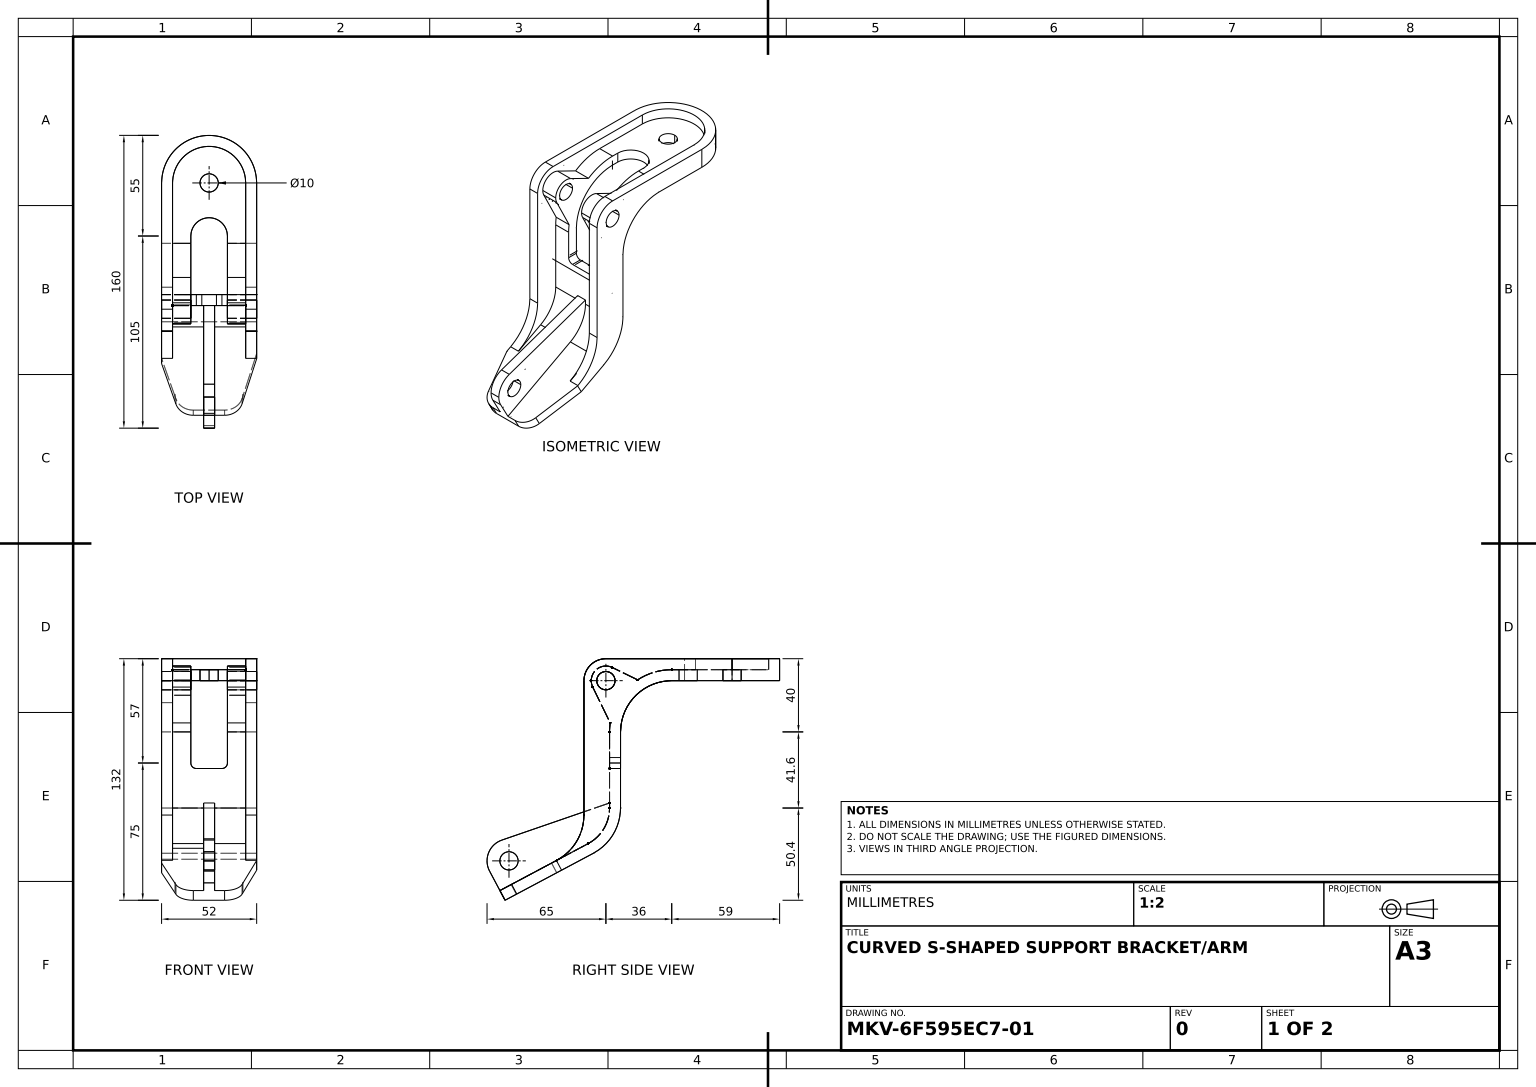
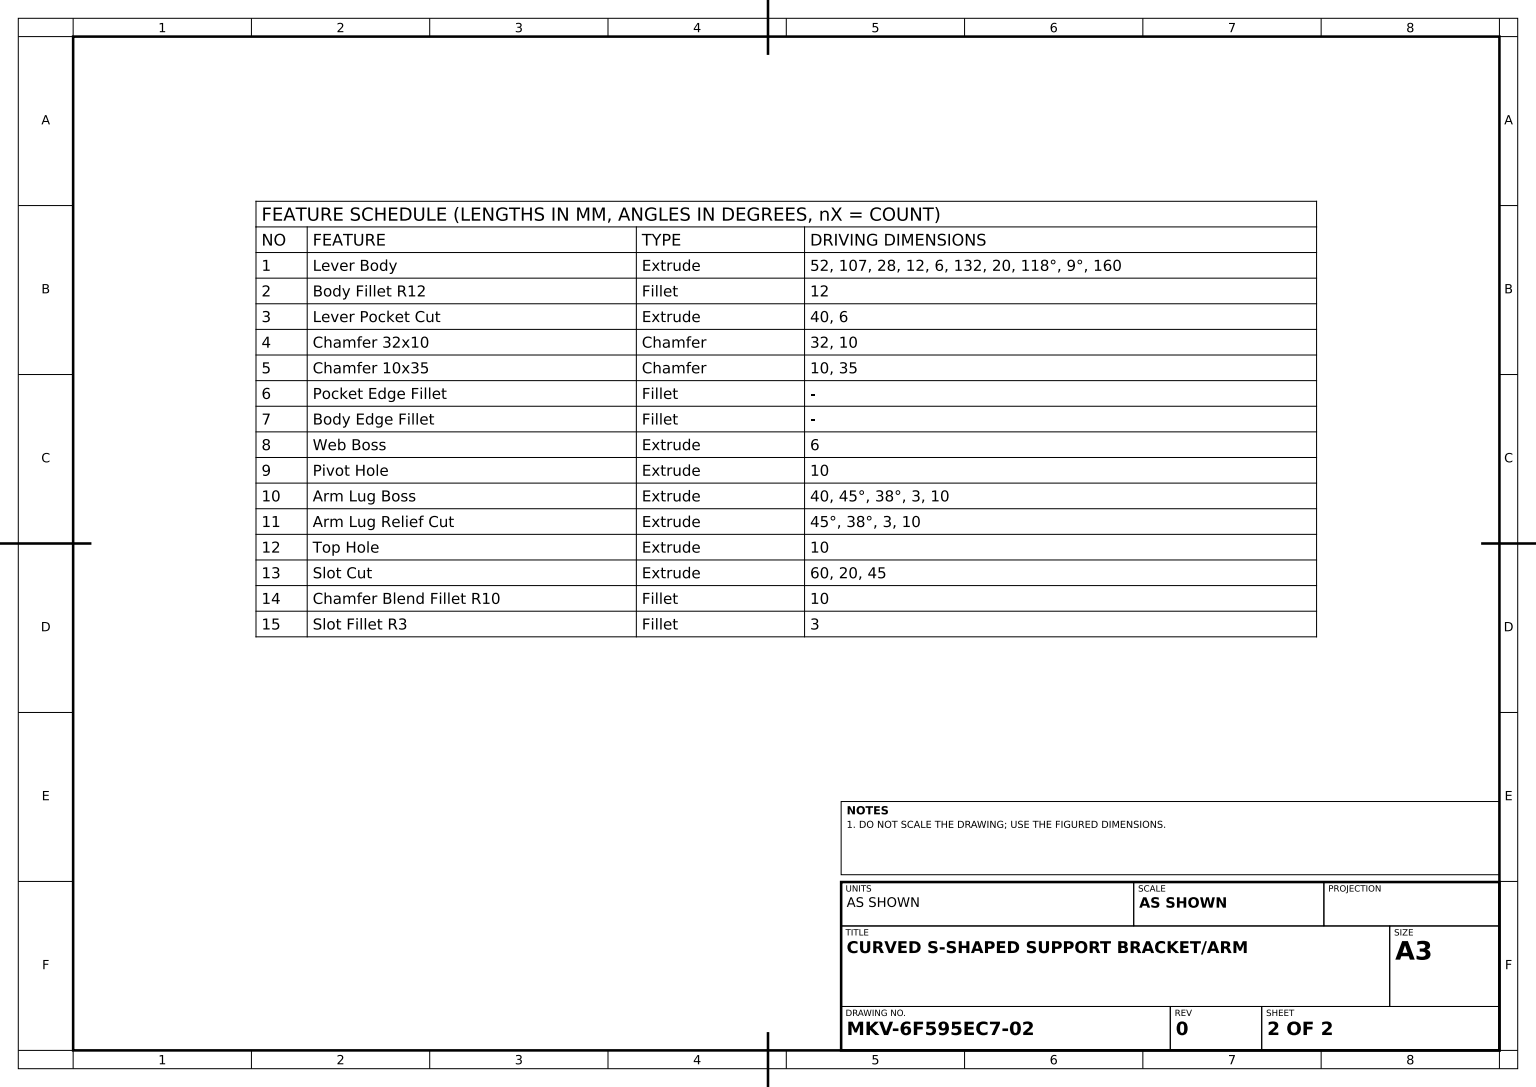
solid
v1 (-3,-110.473285,36)
v2 (3,-110.473285,36)
e1 v1 v2 LINE
v3 (3,-110.473285,46)
e2 v2 v3 CIRCLE(AX(P(3,-110.473285,41),D(1,0,0),D(0,0,-1)),5)
v4 (-3,-110.473285,46)
e3 v4 v3 LINE
e4 v1 v4 CIRCLE(AX(P(-3,-110.473285,41),D(1,0,0),D(0,0,-1)),5)
face CYL(AX(P(-26,-110.473285,41),D(1,0,0),D(0,0,-1)),5) rev [e1 e2 -e3 -e4]
v5 (-3,-99.127062,44.906818)
v6 (-3,-110.473285,53)
e5 v5 v6 CIRCLE(AX(P(-3,-110.473285,41),D(1,0,0),D(0,0,-1)),12)
v7 (3,-110.473285,53)
e6 v7 v6 LINE
v8 (3,-99.127062,44.906818)
e7 v8 v7 CIRCLE(AX(P(3,-110.473285,41),D(1,0,0),D(0,0,-1)),12)
e8 v8 v5 LINE
face CYL(AX(P(3,-110.473285,41),D(-1,0,0),D(0,0,1)),12) [e5 -e6 -e7 e8]
v9 (3,-116.106943,51.595371)
e9 v7 v9 CIRCLE(AX(P(3,-110.473285,41),D(1,0,0),D(0,0,-1)),12)
v10 (3,-126.702314,45.961712)
e10 v9 v10 LINE
v11 (3,-101.02602,-2.328374)
e11 v10 v11 LINE
v12 (3,-81.601173,-14)
e12 v11 v12 CIRCLE(AX(P(3,-81.601173,8),D(1,0,0),D(0,0,-1)),22)
v13 (3,-78.843818,-14)
e13 v12 v13 LINE
e14 v13 v8 LINE
e15 v3 v2 CIRCLE(AX(P(3,-110.473285,41),D(1,0,0),D(0,0,-1)),5)
face PLANE(AX(P(3,-81.601173,8),D(1,0,0),D(0,0,-1))) [e7 e9 e10 e11 e12 e13 e14] [-e15 -e2]
v14 (26,-106.323705,-5.145204)
v15 (-26,-106.323705,-5.145204)
e16 v14 v15 LINE
v16 (-26,-81.601173,-20)
e17 v15 v16 CIRCLE(AX(P(-26,-81.601173,8),D(1,0,0),D(0,0,1)),28)
v17 (26,-81.601173,-20)
e18 v17 v16 LINE
e19 v14 v17 CIRCLE(AX(P(26,-81.601173,8),D(1,0,0),D(0,0,1)),28)
face CYL(AX(P(26,-81.601173,8),D(-1,0,0),D(0,0,1)),28) [e16 e17 -e18 -e19]
v18 (10,-40,-20)
v19 (10,-12,-48)
e20 v18 v19 CIRCLE(AX(P(10,-40,-48),D(-1,0,0),D(0,0,-1)),28)
v20 (26,-12,-48)
e21 v20 v19 LINE
v21 (26,-40,-20)
e22 v21 v20 CIRCLE(AX(P(26,-40,-48),D(-1,0,0),D(0,0,-1)),28)
e23 v21 v18 LINE
face CYL(AX(P(26,-40,-48),D(-1,0,0),D(0,0,1)),28) rev [e20 -e21 -e22 e23]
v22 (26,-85.439941,0)
v23 (20,-85.439941,0)
e24 v22 v23 LINE
v24 (20,-110.162474,14.854796)
e25 v24 v23 CIRCLE(AX(P(20,-85.439941,28),D(1,0,0),D(0,0,-1)),28)
v25 (26,-110.162474,14.854796)
e26 v25 v24 LINE
e27 v22 v25 CIRCLE(AX(P(26,-85.439941,28),D(-1,0,0),D(0,0,-1)),28)
face CYL(AX(P(26,-85.439941,28),D(-1,0,0),D(0,0,1)),28) rev [e24 -e25 -e26 -e27]
v26 (26,0,-81)
v27 (-26,0,-81)
e28 v26 v27 CIRCLE(AX(P(0,0,-81),D(0,1,0),D(0,0,-1)),26)
v28 (-26,0,-12)
e29 v27 v28 LINE
v29 (-20,0,-12)
e30 v28 v29 LINE
v30 (-20,0,-81)
e31 v30 v29 LINE
v31 (20,0,-81)
e32 v31 v30 CIRCLE(AX(P(0,0,-81),D(0,1,0),D(0,0,-1)),20)
v32 (20,0,-12)
e33 v31 v32 LINE
v33 (26,0,-12)
e34 v32 v33 LINE
e35 v26 v33 LINE
face PLANE(AX(P(26,0,0),D(0,-1,0),D(0,0,-1))) rev [e28 e29 e30 -e31 -e32 e33 e34 -e35]
v34 (7,-60,-20)
v35 (-7,-60,-20)
e36 v34 v35 LINE
v36 (-7,-60,-14)
e37 v35 v36 LINE
v37 (7,-60,-14)
e38 v36 v37 LINE
e39 v37 v34 LINE
face PLANE(AX(P(0,-60,-4),D(0,1,0),D(0,0,1))) [e36 e37 e38 e39]
v38 (0,-12,-76)
v39 (0,-6,-76)
e40 v38 v39 LINE
v40 (0,-12,-86)
e41 v40 v38 CIRCLE(AX(P(0,-12,-81),D(0,1,0),D(0,0,1)),5)
v41 (0,-6,-86)
e42 v40 v41 LINE
e43 v39 v41 CIRCLE(AX(P(0,-6,-81),D(0,-1,0),D(0,0,-1)),5)
face CYL(AX(P(0,-132,-81),D(0,1,0),D(0,0,1)),5) rev [-e40 -e41 e42 -e43]
v42 (20,-12,0)
e44 v32 v42 CIRCLE(AX(P(20,-12,-12),D(1,0,0),D(0,0,-1)),12)
v43 (26,-12,0)
e45 v43 v42 LINE
e46 v33 v43 CIRCLE(AX(P(26,-12,-12),D(1,0,0),D(0,0,-1)),12)
face CYL(AX(P(26,-12,-12),D(-1,0,0),D(0,0,1)),12) [e44 -e45 -e46 -e34]
e47 v38 v40 CIRCLE(AX(P(0,-12,-81),D(0,1,0),D(0,0,1)),5)
v44 (26,-12,-81)
e48 v20 v44 LINE
v45 (10,-12,-52)
e49 v19 v45 LINE
v46 (-10,-12,-52)
e50 v45 v46 CIRCLE(AX(P(0,-12,-52),D(0,1,0),D(0,0,1)),10)
v47 (-10,-12,-48)
e51 v47 v46 LINE
v48 (-26,-12,-48)
e52 v47 v48 LINE
v49 (-26,-12,-81)
e53 v48 v49 LINE
e54 v49 v44 CIRCLE(AX(P(0,-12,-81),D(0,-1,0),D(0,0,1)),26)
face PLANE(AX(P(26,-12,-107),D(0,1,0),D(0,0,1))) rev [e47 e41] [-e48 e21 e49 e50 -e51 e52 e53 e54]
e55 v44 v26 LINE
e56 v27 v49 LINE
face CYL(AX(P(0,0,-81),D(0,1,0),D(0,0,1)),26) [-e28 -e55 -e54 -e56]
v50 (10,-6,-52)
e57 v45 v50 LINE
v51 (-10,-6,-52)
e58 v51 v50 CIRCLE(AX(P(0,-6,-52),D(0,-1,0),D(0,0,-1)),10)
e59 v46 v51 LINE
face CYL(AX(P(0,-60,-52),D(0,1,0),D(0,0,1)),10) rev [e57 -e58 -e59 -e50]
v52 (-10,-12,-7)
v53 (-26,-12,-7)
e60 v52 v53 LINE
v54 (-26,-12,-17)
e61 v54 v53 CIRCLE(AX(P(-26,-12,-12),D(1,0,0),D(0,0,-1)),5)
v55 (-10,-12,-17)
e62 v55 v54 LINE
e63 v55 v52 CIRCLE(AX(P(-10,-12,-12),D(1,0,0),D(0,0,-1)),5)
face CYL(AX(P(20,-12,-12),D(-1,0,0),D(0,0,1)),5) rev [e60 -e61 -e62 e63]
v56 (20,-12,-4)
v57 (10,-12,-4)
e64 v56 v57 LINE
v58 (10,-15.506969,-4.809648)
e65 v57 v58 CIRCLE(AX(P(10,-12,-12),D(1,0,0),D(0,0,-1)),8)
v59 (20,-15.506969,-4.809648)
e66 v59 v58 LINE
e67 v56 v59 CIRCLE(AX(P(20,-12,-12),D(1,0,0),D(0,0,-1)),8)
face CYL(AX(P(20,-12,-12),D(-1,0,0),D(0,0,1)),8) [e64 e65 -e66 -e67]
e68 v42 v23 LINE
e69 v43 v22 LINE
face PLANE(AX(P(26,0,0),D(0,0,-1),D(-1,0,0))) rev [e68 -e24 -e69 e45]
e70 v52 v55 CIRCLE(AX(P(-10,-12,-12),D(1,0,0),D(0,0,-1)),5)
e71 v53 v54 CIRCLE(AX(P(-26,-12,-12),D(1,0,0),D(0,0,-1)),5)
face CYL(AX(P(20,-12,-12),D(-1,0,0),D(0,0,1)),5) rev [e70 e62 -e71 -e60]
v60 (-20,-101.02602,-2.328374)
v61 (-20,-81.601173,-14)
e72 v60 v61 CIRCLE(AX(P(-20,-81.601173,8),D(1,0,0),D(0,0,-1)),22)
v62 (-3,-101.02602,-2.328374)
e73 v60 v62 LINE
v63 (-3,-81.601173,-14)
e74 v62 v63 CIRCLE(AX(P(-3,-81.601173,8),D(1,0,0),D(0,0,-1)),22)
e75 v61 v63 LINE
face CYL(AX(P(-20,-81.601173,8),D(1,0,0),D(0,0,-1)),22) rev [-e72 e73 e74 -e75]
v64 (-10,-57,-20)
e76 v64 v35 CIRCLE(AX(P(-7,-57,-20),D(0,0,1),D(0,-1,0)),3)
v65 (10,-57,-20)
e77 v34 v65 CIRCLE(AX(P(7,-57,-20),D(0,0,1),D(0,-1,0)),3)
e78 v65 v18 LINE
e79 v17 v21 LINE
v66 (-26,-40,-20)
e80 v16 v66 LINE
v67 (-10,-40,-20)
e81 v67 v66 LINE
e82 v64 v67 LINE
face PLANE(AX(P(26,-40,-20),D(0,0,1),D(0,-1,0))) rev [e76 -e36 e77 e78 -e23 -e79 e18 e80 -e81 -e82]
v68 (26,-12,-7)
v69 (10,-12,-7)
e83 v68 v69 LINE
v70 (10,-12,-17)
e84 v70 v69 CIRCLE(AX(P(10,-12,-12),D(1,0,0),D(0,0,-1)),5)
v71 (26,-12,-17)
e85 v71 v70 LINE
e86 v71 v68 CIRCLE(AX(P(26,-12,-12),D(1,0,0),D(0,0,-1)),5)
face CYL(AX(P(20,-12,-12),D(-1,0,0),D(0,0,1)),5) rev [e83 -e84 -e85 e86]
e87 v69 v70 CIRCLE(AX(P(10,-12,-12),D(1,0,0),D(0,0,-1)),5)
e88 v68 v71 CIRCLE(AX(P(26,-12,-12),D(1,0,0),D(0,0,-1)),5)
face CYL(AX(P(20,-12,-12),D(-1,0,0),D(0,0,1)),5) rev [-e87 -e83 e88 e85]
e89 v4 v1 CIRCLE(AX(P(-3,-110.473285,41),D(1,0,0),D(0,0,-1)),5)
face CYL(AX(P(-26,-110.473285,41),D(1,0,0),D(0,0,-1)),5) rev [-e1 -e89 e3 e15]
v72 (-10,-11.565692,-29.358913)
v73 (-20,-11.565692,-29.358913)
e90 v72 v73 LINE
v74 (-20,-4.809648,-15.506969)
e91 v73 v74 LINE
v75 (-10,-4.809648,-15.506969)
e92 v75 v74 LINE
e93 v72 v75 LINE
face PLANE(AX(P(20,-4.809648,-15.506969),D(0,-0.898794046,0.438371147),D(0,-0.438371147,-0.898794046))) rev [e90 e91 -e92 -e93]
v76 (10,-11.565692,-29.358913)
v77 (10,-4.809648,-15.506969)
e94 v76 v77 LINE
v78 (10,-6,-48)
e95 v76 v78 CIRCLE(AX(P(10,-40,-48),D(-1,0,0),D(0,0,-1)),34)
e96 v50 v78 LINE
v79 (10,-57,-14)
e97 v65 v79 LINE
v80 (10,-40,-14)
e98 v80 v79 LINE
v81 (10,-35.082851,-14.357443)
e99 v80 v81 CIRCLE(AX(P(10,-40,-48),D(-1,0,0),D(0,0,-1)),34)
e100 v58 v81 LINE
e101 v77 v57 CIRCLE(AX(P(10,-12,-12),D(1,0,0),D(0,0,-1)),8)
face PLANE(AX(P(10,-60,-4),D(1,0,0),D(0,0,-1))) rev [e84 e87] [-e94 e95 -e96 -e57 -e49 -e20 -e78 e97 -e98 e99 -e100 -e65 -e101]
v82 (-20,-15.506969,-4.809648)
v83 (-20,-35.082851,-14.357443)
e102 v82 v83 LINE
v84 (-10,-35.082851,-14.357443)
e103 v84 v83 LINE
v85 (-10,-15.506969,-4.809648)
e104 v85 v84 LINE
e105 v85 v82 LINE
face PLANE(AX(P(20,-15.506969,-4.809648),D(0,0.438371147,-0.898794046),D(0,0.898794046,0.438371147))) rev [e102 -e103 -e104 e105]
e106 v66 v48 CIRCLE(AX(P(-26,-40,-48),D(-1,0,0),D(0,0,-1)),28)
v86 (-26,-116.97691,14.89056)
e107 v86 v15 LINE
v87 (-26,-111.679224,17.707389)
e108 v86 v87 LINE
v88 (-26,-110.162474,14.854796)
e109 v88 v87 LINE
v89 (-26,-85.439941,0)
e110 v89 v88 CIRCLE(AX(P(-26,-85.439941,28),D(-1,0,0),D(0,0,-1)),28)
v90 (-26,-12,0)
e111 v90 v89 LINE
e112 v90 v28 CIRCLE(AX(P(-26,-12,-12),D(-1,0,0),D(0,0,-1)),12)
face PLANE(AX(P(-26,-85.439941,28),D(1,0,0),D(0,0,-1))) rev [-e29 e56 -e53 -e106 -e80 -e17 -e107 e108 -e109 -e110 -e111 e112] [e61 e71]
v91 (20,-4.809648,-15.506969)
e113 v91 v56 CIRCLE(AX(P(20,-12,-12),D(1,0,0),D(0,0,-1)),8)
e114 v91 v77 LINE
face CYL(AX(P(20,-12,-12),D(-1,0,0),D(0,0,1)),8) [-e64 -e113 e114 e101]
v92 (18.072225,-128.595022,36.741051)
v93 (8.456986,-132,43.144883)
e115 v92 v93 CIRCLE(AX(P(8.456986,-127.305284,34.315407),D(0,-0.882947593,-0.469471563),D(0,-0.469471563,0.882947593)),10)
v94 (18.072225,-123.297336,39.55788)
e116 v94 v92 LINE
v95 (8.456986,-126.702314,45.961712)
e117 v95 v94 CIRCLE(AX(P(8.456986,-122.007599,37.132236),D(0,0.882947593,0.469471563),D(0,0.469471563,-0.882947593)),10)
e118 v93 v95 LINE
face CYL(AX(P(8.456986,-127.305284,34.315407),D(0,-0.882947593,-0.469471563),D(0,0.469471563,-0.882947593)),10) [-e115 -e116 -e117 -e118]
v96 (-20,-110.162474,14.854796)
e119 v60 v96 LINE
e120 v96 v88 LINE
v97 (-18.192891,-123.407915,39.765848)
e121 v87 v97 LINE
v98 (-8.648091,-126.702314,45.961712)
e122 v97 v98 CIRCLE(AX(P(-8.648091,-122.007599,37.132236),D(0,0.882947593,0.469471563),D(0,0.469471563,-0.882947593)),10)
v99 (-3,-126.702314,45.961712)
e123 v99 v98 LINE
e124 v99 v62 LINE
face PLANE(AX(P(26,-126.702314,45.961712),D(0,-0.882947593,-0.469471563),D(0,0.469471563,-0.882947593))) rev [e119 e120 e109 e121 e122 -e123 e124 -e73]
v100 (-20,-12,-4)
e125 v74 v100 CIRCLE(AX(P(-20,-12,-12),D(1,0,0),D(0,0,-1)),8)
v101 (-10,-12,-4)
e126 v101 v100 LINE
e127 v75 v101 CIRCLE(AX(P(-10,-12,-12),D(1,0,0),D(0,0,-1)),8)
face CYL(AX(P(20,-12,-12),D(-1,0,0),D(0,0,1)),8) [e125 -e126 -e127 e92]
v102 (26,-110.27081,15.058547)
v103 (26,-115.568495,12.241717)
e128 v102 v103 LINE
e129 v94 v102 LINE
e130 v103 v92 LINE
face PLANE(AX(P(26,-85.548277,28.20375),D(0.961523948,-0.128973757,0.242564359),D(0,0.882947593,0.469471563))) [-e128 -e129 e116 -e130]
e131 v67 v47 CIRCLE(AX(P(-10,-40,-48),D(-1,0,0),D(0,0,-1)),28)
face CYL(AX(P(26,-40,-48),D(-1,0,0),D(0,0,1)),28) rev [-e52 -e131 e81 e106]
v104 (-3,-78.843818,-14)
e132 v13 v104 LINE
e133 v104 v5 LINE
face PLANE(AX(P(3,-99.127062,44.906818),D(0,-0.945518576,-0.325568154),D(0,0.325568154,-0.945518576))) rev [-e8 -e14 e132 e133]
v105 (-18.192891,-128.705601,36.949019)
e134 v105 v97 LINE
e135 v105 v86 LINE
face PLANE(AX(P(-16,-132,43.144883),D(0.954479978,0.140031627,-0.263361187),D(0,-0.882947593,-0.469471563))) rev [e134 -e121 -e108 -e135]
v106 (-3,-116.106943,51.595371)
e136 v6 v106 CIRCLE(AX(P(-3,-110.473285,41),D(1,0,0),D(0,0,-1)),12)
e137 v9 v106 LINE
face CYL(AX(P(3,-110.473285,41),D(-1,0,0),D(0,0,1)),12) [e6 e136 -e137 -e9]
v107 (-20,-40,-14)
e138 v83 v107 CIRCLE(AX(P(-20,-40,-48),D(1,0,0),D(0,0,-1)),34)
v108 (-10,-40,-14)
e139 v107 v108 LINE
e140 v108 v84 CIRCLE(AX(P(-10,-40,-48),D(-1,0,0),D(0,0,-1)),34)
face CYL(AX(P(-20,-40,-48),D(1,0,0),D(0,0,-1)),34) [e138 e139 e140 e103]
e141 v106 v99 LINE
v109 (-8.648091,-132,43.144883)
e142 v98 v109 LINE
e143 v93 v109 LINE
e144 v95 v10 LINE
face PLANE(AX(P(26,-132,43.144883),D(0,0.469471563,-0.882947593),D(0,0.882947593,0.469471563))) rev [e141 e123 e142 -e143 e118 e144 -e10 e137]
e145 v109 v105 CIRCLE(AX(P(-8.648091,-127.305284,34.315407),D(0,-0.882947593,-0.469471563),D(0,-0.469471563,0.882947593)),10)
face CYL(AX(P(-8.648091,-127.305284,34.315407),D(0,-0.882947593,-0.469471563),D(0,0.469471563,-0.882947593)),10) [-e122 -e134 -e145 -e142]
v110 (-10,-6,-48)
e146 v72 v110 CIRCLE(AX(P(-10,-40,-48),D(-1,0,0),D(0,0,-1)),34)
v111 (-20,-6,-48)
e147 v111 v110 LINE
e148 v111 v73 CIRCLE(AX(P(-20,-40,-48),D(1,0,0),D(0,0,-1)),34)
face CYL(AX(P(-20,-40,-48),D(1,0,0),D(0,0,-1)),34) [-e90 e146 -e147 e148]
e149 v63 v104 LINE
v112 (20,-81.601173,-14)
e150 v12 v112 LINE
v113 (20,-40,-14)
e151 v112 v113 LINE
e152 v80 v113 LINE
e153 v79 v37 CIRCLE(AX(P(7,-57,-14),D(0,0,-1),D(0,1,0)),3)
v114 (-10,-57,-14)
e154 v36 v114 CIRCLE(AX(P(-7,-57,-14),D(0,0,-1),D(0,1,0)),3)
e155 v108 v114 LINE
e156 v61 v107 LINE
face PLANE(AX(P(-20,-81.601173,-14),D(0,0,-1),D(0,1,0))) rev [e75 e149 -e132 -e13 e150 e151 -e152 e98 e153 -e38 e154 -e155 -e139 -e156]
e157 v41 v39 CIRCLE(AX(P(0,-6,-81),D(0,-1,0),D(0,0,-1)),5)
e158 v51 v110 LINE
v115 (20,-6,-48)
e159 v78 v115 LINE
v116 (20,-6,-81)
e160 v115 v116 LINE
v117 (-20,-6,-81)
e161 v116 v117 CIRCLE(AX(P(0,-6,-81),D(0,1,0),D(0,0,-1)),20)
e162 v111 v117 LINE
face PLANE(AX(P(-20,-6,-48),D(0,-1,0),D(0,0,-1))) rev [e43 e157] [-e158 e58 e96 e159 e160 e161 -e162 e147]
v118 (20,-35.082851,-14.357443)
e163 v118 v81 LINE
e164 v59 v118 LINE
face PLANE(AX(P(20,-15.506969,-4.809648),D(0,0.438371147,-0.898794046),D(0,0.898794046,0.438371147))) rev [e100 -e163 -e164 e66]
e165 v117 v30 LINE
v119 (-20,-12,0)
e166 v29 v119 CIRCLE(AX(P(-20,-12,-12),D(1,0,0),D(0,0,-1)),12)
v120 (-20,-85.439941,0)
e167 v119 v120 LINE
e168 v96 v120 CIRCLE(AX(P(-20,-85.439941,28),D(1,0,0),D(0,0,-1)),28)
e169 v100 v82 CIRCLE(AX(P(-20,-12,-12),D(1,0,0),D(0,0,-1)),8)
face PLANE(AX(P(-20,-12,-12),D(1,0,0),D(0,0,-1))) [-e125 -e91 -e148 e162 e165 e31 e166 e167 -e168 -e119 e72 e156 -e138 -e102 -e169]
e170 v101 v85 CIRCLE(AX(P(-10,-12,-12),D(1,0,0),D(0,0,-1)),8)
e171 v114 v64 LINE
face PLANE(AX(P(-10,-60,-4),D(1,0,0),D(0,0,-1))) [e158 -e146 e93 e127 e170 e104 -e140 e155 e171 e82 e131 e51 e59] [-e63 -e70]
v121 (20,-11.565692,-29.358913)
e172 v121 v76 LINE
e173 v115 v121 CIRCLE(AX(P(20,-40,-48),D(1,0,0),D(0,0,-1)),34)
face CYL(AX(P(-20,-40,-48),D(1,0,0),D(0,0,-1)),34) [-e95 -e172 -e173 -e159]
v122 (20,-101.02602,-2.328374)
e174 v122 v112 CIRCLE(AX(P(20,-81.601173,8),D(1,0,0),D(0,0,-1)),22)
e175 v11 v122 LINE
face CYL(AX(P(-20,-81.601173,8),D(1,0,0),D(0,0,-1)),22) rev [e174 -e150 -e12 e175]
e176 v118 v113 CIRCLE(AX(P(20,-40,-48),D(1,0,0),D(0,0,-1)),34)
face CYL(AX(P(-20,-40,-48),D(1,0,0),D(0,0,-1)),34) [-e176 e163 -e99 e152]
e177 v31 v116 LINE
face CYL(AX(P(0,-6,-81),D(0,1,0),D(0,0,1)),20) rev [-e161 -e177 e32 -e165]
e178 v120 v89 LINE
e179 v119 v90 LINE
face PLANE(AX(P(26,0,0),D(0,0,-1),D(-1,0,0))) rev [-e178 -e167 e179 e111]
face CYL(AX(P(26,-85.439941,28),D(-1,0,0),D(0,0,1)),28) rev [-e120 e168 e178 e110]
face CYL(AX(P(0,-132,-81),D(0,1,0),D(0,0,1)),5) rev [e40 -e157 -e42 -e47]
face CYL(AX(P(20,-12,-12),D(-1,0,0),D(0,0,1)),8) [e169 -e105 -e170 e126]
e180 v25 v102 LINE
e181 v122 v24 LINE
face PLANE(AX(P(26,-126.702314,45.961712),D(0,-0.882947593,-0.469471563),D(0,0.469471563,-0.882947593))) rev [-e175 -e11 -e144 e117 e129 -e180 e26 -e181]
face CYL(AX(P(26,-12,-12),D(-1,0,0),D(0,0,1)),12) [-e30 -e112 -e179 -e166]
e182 v103 v14 LINE
face PLANE(AX(P(26,-85.439941,28),D(1,0,0),D(0,0,-1))) [-e88 -e86] [e55 e35 e46 e69 e27 e180 e128 e182 e19 e79 e22 e48]
e183 v121 v91 LINE
face PLANE(AX(P(20,-12,-12),D(1,0,0),D(0,0,-1))) rev [e164 e176 -e151 -e174 e181 e25 -e68 -e44 -e33 e177 -e160 e173 e183 e113 e67]
face CYL(AX(P(-7,-57,-4),D(0,0,1),D(1,0,0)),3) rev [-e171 -e154 -e37 -e76]
face PLANE(AX(P(26,-106.323705,-5.145204),D(0,0.882947593,0.469471563),D(0,-0.469471563,0.882947593))) rev [e143 e145 e135 e107 -e16 -e182 e130 e115]
face CYL(AX(P(7,-57,-4),D(0,0,-1),D(-1,0,0)),3) rev [-e153 -e97 -e77 -e39]
face PLANE(AX(P(20,-4.809648,-15.506969),D(0,-0.898794046,0.438371147),D(0,-0.438371147,-0.898794046))) rev [-e183 e172 e94 -e114]
face PLANE(AX(P(-3,-81.601173,8),D(1,0,0),D(0,0,-1))) rev [e89 e4] [-e133 -e149 -e74 -e124 -e141 -e136 -e5]
